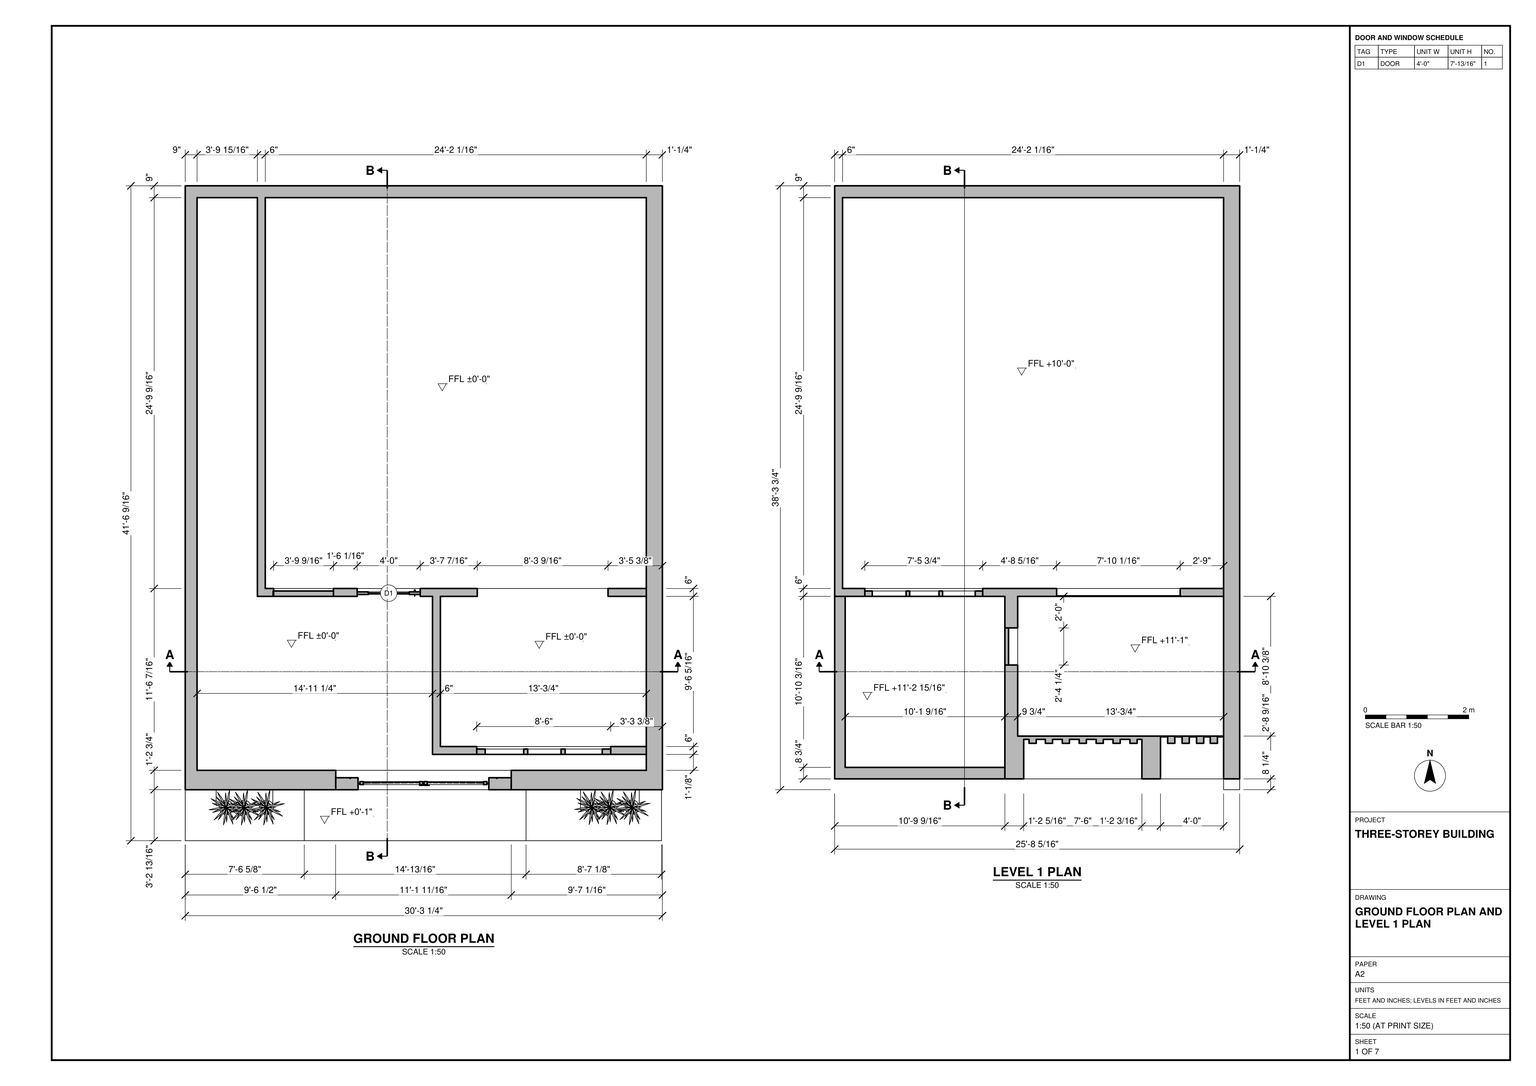
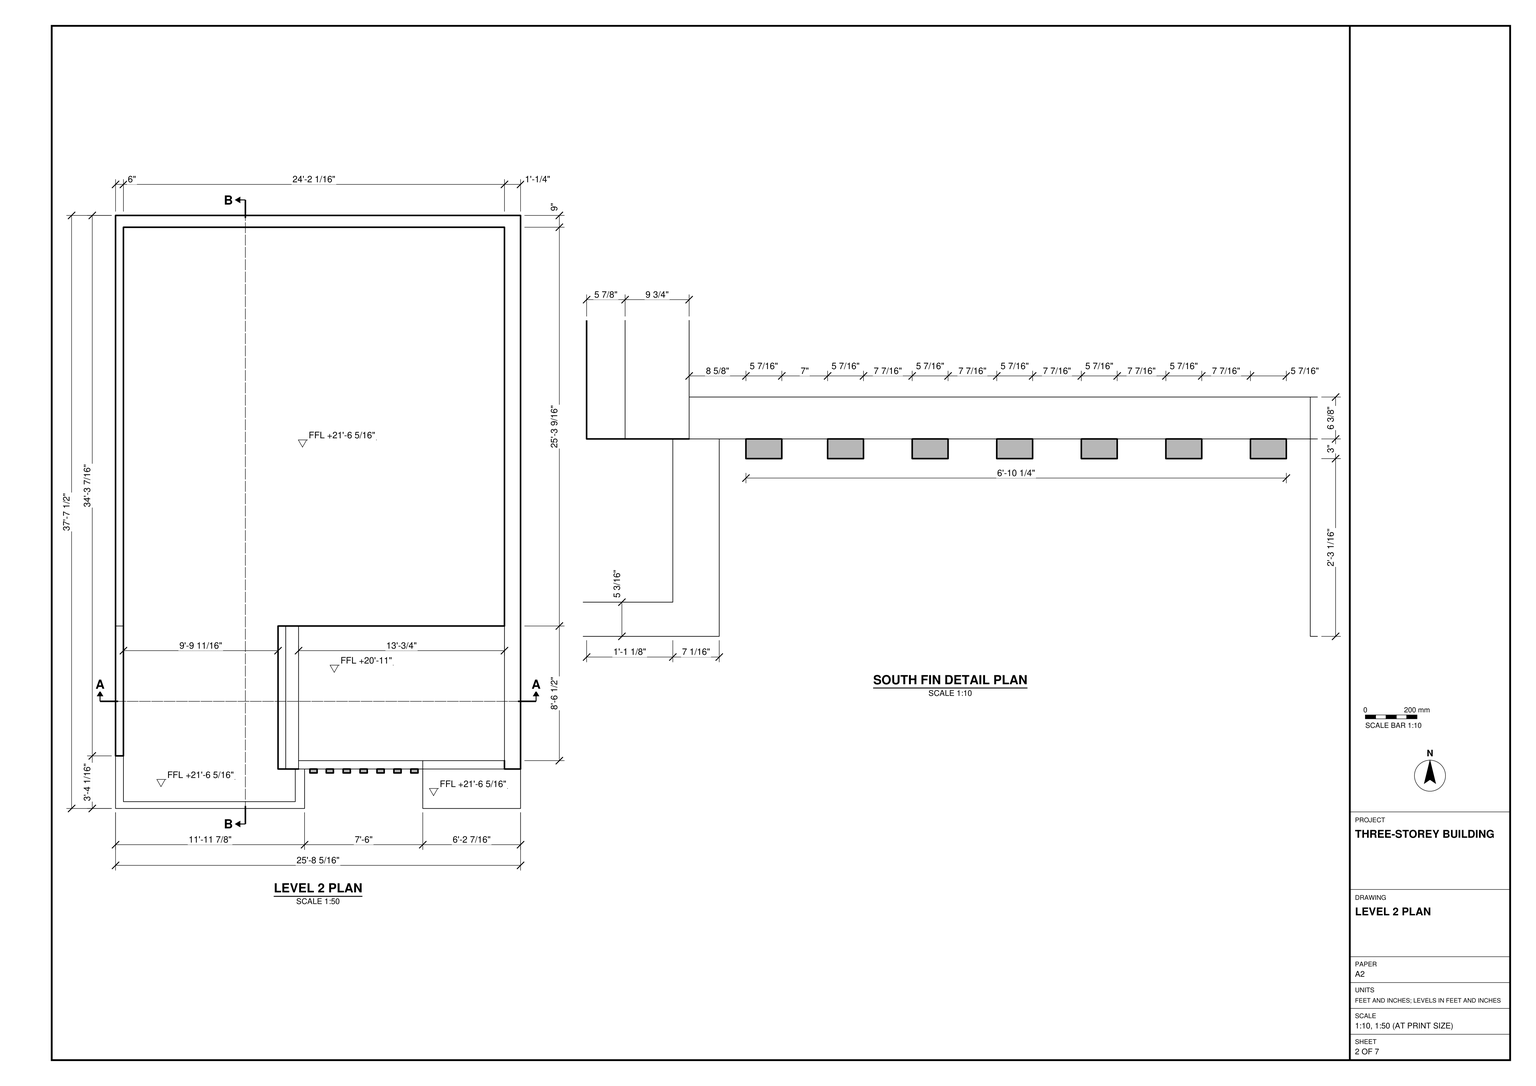
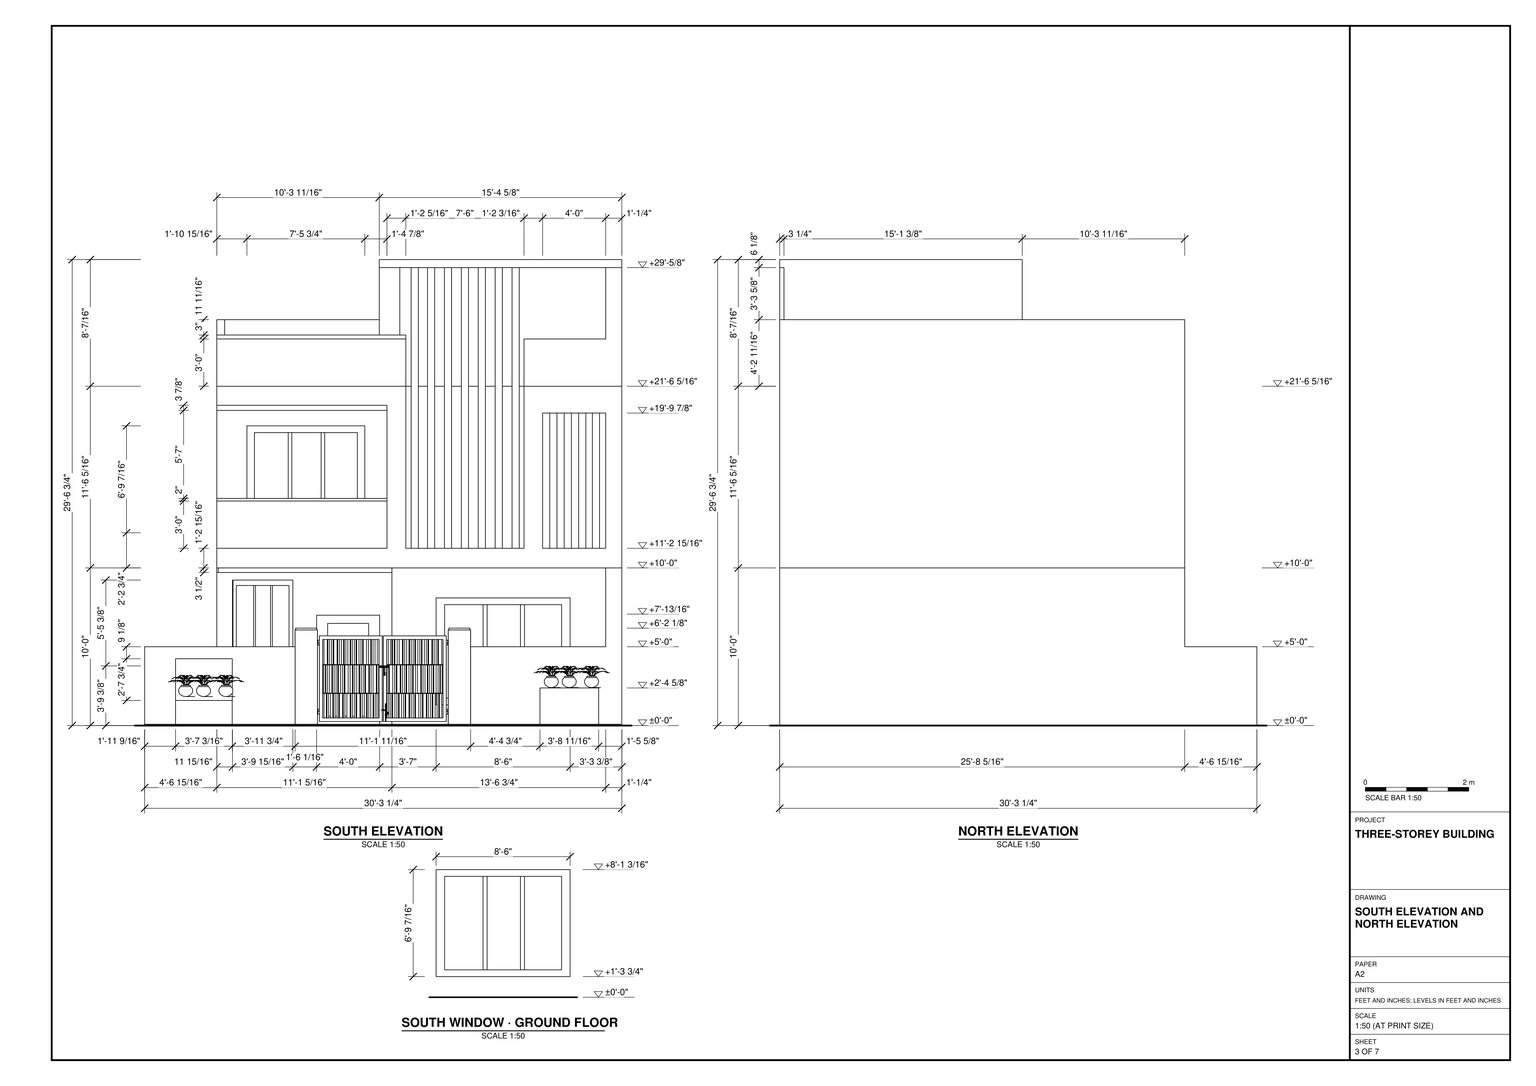
Build the three-storey building in SketchUp from task_files/diagram_01.pdf. Work in feet and inches. The overall model is 30'-3 1/4" wide, 41'-6 9/16" deep and 29'-6 3/4" high. Set the principal levels at ±0'-0", +10'-0" and +21'-6 5/16". Use the local floor levels on the plans for the areas that sit above or below these principal levels.

Lay out the ground-floor enclosure, including the narrow strip along the west side and the front room set back from the south boundary wall. Build the perimeter walls and partitions at their drawn thicknesses. Follow the upper plans for the narrower building footprint, floor slabs, roof and parapets. On the south face, place the framed openings behind the boundary wall and model the double-leaf entrance gate between its piers. Reproduce the recessed upper opening, the stepped roofline and the two fields of vertical fins. Use the fin detail plan to set the spacing and projection of the blades. Place the front planting on either side of the gate. Decor and loose items, including plants, may be any suitable library components.

Keep shell elements such as walls, slabs and roof, and each furniture or joinery piece shown, in separate groups or components. Use components for repeated parts. Save one SketchUp model as output_files/three_storey_building_with_a_finned_south_facade.skp.

# SketchUp Ruby script. Lengths in inches.
U = 1.inch
M = Sketchup.active_model
def pt(a) = Geom::Point3d.new(a.map { |v| v * U })
def face(e, loops, mat)
  f = e.add_face(loops[0].map { |a| pt(a) })
  loops[1..].each { |l| e.add_face(l.map { |a| pt(a) }).erase! }
  f.material = f.back_material = mat if mat
  f
end
# faces: each face lists its corners as indices into pts; further lists are holes
def faces(e, pts, list, mat = nil) = list.each { |f| face(e, (f[0].is_a?(Array) ? f : [f]).map { |l| l.map { |i| pts[i] } }, mat) }
# xy, xz, yz: faces in a plane at the given z, y or x. An outline is a flat list of corners, or four numbers for a rectangle; further outlines are holes
def ring(l) = l.size == 4 ? [[l[0], l[1]], [l[2], l[1]], [l[2], l[3]], [l[0], l[3]]] : l.each_slice(2).to_a
def flat(e, list, mat, &to3) = list.each { |f| face(e, (f[0].is_a?(Array) ? f : [f]).map { |l| ring(l).map { |u, v| to3.(u, v) } }, mat) }
def xy(e, z, list, mat = nil) = flat(e, list, mat) { |x, y| [x, y, z] }
def xz(e, y, list, mat = nil) = flat(e, list, mat) { |x, z| [x, y, z] }
def yz(e, x, list, mat = nil) = flat(e, list, mat) { |y, z| [x, y, z] }
def lines(e, pts, list) = list.each { |a, b| e.add_line(pt(pts[a]), pt(pts[b])) }
# prism: a flat outline (further loops are holes) pulled along v
def prism(e, loops, v, mat = nil)
  f = face(e, loops, mat); d = Geom::Vector3d.new(v.map { |x| x * U })
  f.pushpull(f.normal.samedirection?(d) ? d.length : -d.length)
end
def box(e, o, s, mat = nil) = prism(e, [[o, [o[0] + s[0], o[1], o[2]], [o[0] + s[0], o[1] + s[1], o[2]], [o[0], o[1] + s[1], o[2]]]], [0, 0, s[2]], mat)
def at(x, y, z, deg = 0) = Geom::Transformation.translation(pt([x, y, z])) * Geom::Transformation.rotation(ORIGIN, Z_AXIS, deg.degrees)
def axes(o, x, y, z) = Geom::Transformation.new([*x, 0, *y, 0, *z, 0, *pt(o).to_a, 1])
def part(name) = M.definitions.add(name)
# library, detail: a bought-in or finely detailed component or shape, given as its bounding box
def library(name, o, s) = part(name).tap { |d| box(d.entities, o, s) }
def detail(e, o, s) = box(e.add_group.entities, o, s)
def put(e, d, t, mat = nil) = e.add_instance(d, t).tap { |i| i.material = mat if mat }
def group(e, t, mat = nil) = e.add_group.tap { |g| g.transformation = t; g.material = mat if mat }.entities
root = M.entities
M.materials.add("3064d055d501e5e6b0f6546dbac280ca7b3e63756ead2-EpHpDy_fw4").color = [149, 120, 88]
M.materials.add("[Blacktop Old 02]").color = [143, 145, 145]
M.materials.add("[Blinds Roman Hobbled Blue]").color = [81, 82, 87]
M.materials.add("[Brick Tumbled]").color = [135, 132, 132]
M.materials.add("[Color C08]").color = [102, 51, 0]
M.materials.add("[Color H07]").color = [0, 153, 153]
M.materials.add("[Color L06]").color = [204, 0, 100]
M.materials.add("[Color L16]").color = [102, 0, 51]
M.materials.add("[Concrete Aggregate Smoke]").color = [154, 150, 148]
M.materials.add("[Concrete Form 4x8]").color = [167, 170, 168]
M.materials.add("[Grass Dark Green]").color = [106, 157, 55]
M.materials.add("[Metal Seamed]").color = [118, 119, 115]
M.materials.add("[Stone Flagstone Ashlar]").color = [175, 116, 102]
M.materials.add("[Translucent Glass Gray]").color = [128, 128, 128]
M.materials["[Translucent Glass Gray]"].alpha = 0.5
M.materials.add("[Wood Veneer 01]").color = [120, 70, 37]
c1 = library("Glass Door",[128.54,164.83,0],[40,4.88,84.84])
c2 = library("组\#1607",[0,0,0],[105.03,15.75,105.99])
c3 = part("组\#1597")
box(c3.entities,[0,0,0],[9.65,0.39,1.97])
box(c3.entities,[10.43,0,0],[1.58,0.39,1.97])
c4 = part("组\#1599")
prism(c4.entities,[[[0.05,0.59,0],[0.12,0.67,0],[0.2,0.73,0],[0.29,0.77,0],[0.39,0.79,0],[0.5,0.77,0],[0.59,0.73,0],[0.67,0.67,0],[0.73,0.59,0],[0.77,0.5,0],[0.79,0.39,0],[0.77,0.29,0],[0.73,0.2,0],[0.67,0.12,0],[0.59,0.05,0],[0.5,0.01,0],[0.39,0,0],[0.29,0.01,0],[0.2,0.05,0],[0.12,0.12,0],[0.05,0.2,0],[0.01,0.29,0],[0,0.39,0],[0.01,0.5,0]]],[0,0,12.4])
c5 = part("组\#1598")
prism(c5.entities,[[[-0.39,1.18,0.59],[-0.39,1.16,0.4375],[-0.39,1.1,0.3],[-0.39,1.01,0.17],[-0.39,0.89,0.08],[-0.39,0.74,0.02],[-0.39,0.59,0],[-0.39,0.4375,0.02],[-0.39,0.3,0.08],[-0.39,0.17,0.17],[-0.39,0.08,0.3],[-0.39,0.02,0.4375],[-0.39,0,0.59],[-0.39,0.02,0.74],[-0.39,0.08,0.89],[-0.39,0.17,1.01],[-0.39,0.3,1.1],[-0.39,0.4375,1.16],[-0.39,0.59,1.18],[-0.39,0.74,1.16],[-0.39,0.89,1.1],[-0.39,1.01,1.01],[-0.39,1.1,0.89],[-0.39,1.16,0.74]],[[-0.39,0.98,0.59],[-0.39,0.97,0.69],[-0.39,0.93,0.79],[-0.39,0.87,0.87],[-0.39,0.79,0.93],[-0.39,0.69,0.97],[-0.39,0.59,0.98],[-0.39,0.49,0.97],[-0.39,0.39,0.93],[-0.39,0.3125,0.87],[-0.39,0.25,0.79],[-0.39,0.21,0.69],[-0.39,0.2,0.59],[-0.39,0.21,0.49],[-0.39,0.25,0.39],[-0.39,0.3125,0.3125],[-0.39,0.39,0.25],[-0.39,0.49,0.21],[-0.39,0.59,0.2],[-0.39,0.69,0.21],[-0.39,0.79,0.25],[-0.39,0.87,0.3125],[-0.39,0.93,0.39],[-0.39,0.97,0.49]]],[1.97,0,0])
c6 = part("组\#1600")
prism(c6.entities,[[[0,1.18,0.59],[0,1.16,0.4375],[0,1.1,0.3],[0,1.01,0.17],[0,0.89,0.08],[0,0.74,0.02],[0,0.59,0],[0,0.4375,0.02],[0,0.3,0.08],[0,0.17,0.17],[0,0.08,0.3],[0,0.02,0.4375],[0,0,0.59],[0,0.02,0.74],[0,0.08,0.89],[0,0.17,1.01],[0,0.3,1.1],[0,0.4375,1.16],[0,0.59,1.18],[0,0.74,1.16],[0,0.89,1.1],[0,1.01,1.01],[0,1.1,0.89],[0,1.16,0.74]],[[0,0.98,0.59],[0,0.97,0.69],[0,0.93,0.79],[0,0.87,0.87],[0,0.79,0.93],[0,0.69,0.97],[0,0.59,0.98],[0,0.49,0.97],[0,0.39,0.93],[0,0.3125,0.87],[0,0.25,0.79],[0,0.21,0.69],[0,0.2,0.59],[0,0.21,0.49],[0,0.25,0.39],[0,0.3125,0.3125],[0,0.39,0.25],[0,0.49,0.21],[0,0.59,0.2],[0,0.69,0.21],[0,0.79,0.25],[0,0.87,0.3125],[0,0.93,0.39],[0,0.97,0.49]]],[1.18,0,0])
c7 = part("组\#1601")
prism(c7.entities,[[[0,1.18,0.59],[0,1.16,0.4375],[0,1.1,0.3],[0,1.01,0.17],[0,0.89,0.08],[0,0.74,0.02],[0,0.59,0],[0,0.4375,0.02],[0,0.3,0.08],[0,0.17,0.17],[0,0.08,0.3],[0,0.02,0.4375],[0,0,0.59],[0,0.02,0.74],[0,0.08,0.89],[0,0.17,1.01],[0,0.3,1.1],[0,0.4375,1.16],[0,0.59,1.18],[0,0.74,1.16],[0,0.89,1.1],[0,1.01,1.01],[0,1.1,0.89],[0,1.16,0.74]],[[0,0.98,0.59],[0,0.97,0.69],[0,0.93,0.79],[0,0.87,0.87],[0,0.79,0.93],[0,0.69,0.97],[0,0.59,0.98],[0,0.49,0.97],[0,0.39,0.93],[0,0.3125,0.87],[0,0.25,0.79],[0,0.21,0.69],[0,0.2,0.59],[0,0.21,0.49],[0,0.25,0.39],[0,0.3125,0.3125],[0,0.39,0.25],[0,0.49,0.21],[0,0.59,0.2],[0,0.69,0.21],[0,0.79,0.25],[0,0.87,0.3125],[0,0.93,0.39],[0,0.97,0.49]]],[1.57,0,0])
c8 = part("组\#1591")
xy(c8.entities,0,[[0.12,0,1.0625,0.39]])
xy(c8.entities,0.39,[[0,0,1.18,0.39]])
xy(c8.entities,0.79,[[0.39,0,0.79,0.39]])
xy(c8.entities,2.36,[[0.39,0,0.79,0.39]])
xy(c8.entities,2.76,[[0,0,1.18,0.39]])
xy(c8.entities,9.84,[[0,0,1.18,0.39]])
xz(c8.entities,0,[[0.12,0,1.0625,0,1.18,0.12,1.18,0.39,0,0.39,0,0.12],[[0,0.39,1.18,2.76],[0.39,0.79,0.79,2.36]],[0,2.76,1.18,9.84]])
xz(c8.entities,0.39,[[0.12,0,0,0.12,0,0.39,1.18,0.39,1.18,0.12,1.0625,0],[[0,0.39,1.18,2.76],[0.39,0.79,0.79,2.36]],[0,2.76,1.18,9.84]])
yz(c8.entities,0,[[0,0.12,0.39,0.39],[0,0.39,0.39,2.76],[0,2.76,0.39,8.46],[0,8.46,0.39,9.06],[0,9.06,0.39,9.84]])
yz(c8.entities,0.39,[[0,0.79,0.39,2.36]])
yz(c8.entities,0.79,[[0,0.79,0.39,2.36]])
yz(c8.entities,1.18,[[0,0.12,0.39,0.39],[0,0.39,0.39,2.76],[0,2.76,0.39,8.46],[0,8.46,0.39,8.86],[0,8.86,0.39,9.84]])
p = [[0.12,0,0],[0,0,0.12],[0,0.39,0.12],[0.12,0.39,0],[1.18,0,0.12],[1.0625,0,0],
  [1.0625,0.39,0],[1.18,0.39,0.12]]
faces(c8.entities,p,[[0,1,2,3],[4,5,6,7]])
c9 = part("组\#1592")
xy(c9.entities,0,[[0,0.71,0.8,1.1],[0.8,0.71,1.98,1.1],[1.98,0.71,3.95,1.1]])
xy(c9.entities,0.39,[[1.19,-0.63,1.59,1.1]])
xy(c9.entities,1.97,[[1.19,-0.63,1.59,1.1]])
xy(c9.entities,2.36,[[0,0.71,0.8,1.1],[0.8,0.71,1.98,1.1],[1.98,0.71,3.95,1.1]])
xz(c9.entities,-0.63,[[1.19,0.39,1.59,1.97]])
xz(c9.entities,0.71,[[0,0,3.95,2.36]])
xz(c9.entities,1.1,[[0,0,0.8,2.36],[[0.8,0,1.98,2.36],[1.19,0.39,1.59,1.97]],[1.98,0,3.95,2.36]])
yz(c9.entities,0,[[0.71,0,1.1,2.36]])
yz(c9.entities,1.19,[[-0.63,0.39,1.1,1.97]])
yz(c9.entities,1.59,[[-0.63,0.39,1.1,1.97]])
yz(c9.entities,3.95,[[0.71,0,1.1,2.36]])
c10 = part("组\#1602")
put(c10.entities,c8,at(0.8,0.39,0))
put(c10.entities,c9,at(-0.04,0.43,0.39))
c11 = part("组\#1609")
put(c11.entities,c3,at(0,1.1875,8.46))
put(c11.entities,c4,axes([0,0.2,9.84],[0,0,-1],[0,1,0],[1,0,0]))
put(c11.entities,c5,at(8.07,0.01,8.86))
put(c11.entities,c6,at(1.77,0.01,8.86))
put(c11.entities,c7,at(10.43,0.01,8.86))
put(c11.entities,c10,at(5.7,0,-0.16))
c12 = part("组\#1604")
prism(c12.entities,[[[0.08,0.89,0],[0.17,1.01,0],[0.3,1.1,0],[0.4375,1.16,0],[0.59,1.18,0],[0.74,1.16,0],[0.89,1.1,0],[1.01,1.01,0],[1.1,0.89,0],[1.16,0.74,0],[1.18,0.59,0],[1.16,0.4375,0],[1.1,0.3,0],[1.01,0.17,0],[0.89,0.08,0],[0.74,0.02,0],[0.59,0,0],[0.4375,0.02,0],[0.3,0.08,0],[0.17,0.17,0],[0.08,0.3,0],[0.02,0.4375,0],[0,0.59,0],[0.02,0.74,0]],[[0.97,0.49,0],[0.98,0.59,0],[0.97,0.69,0],[0.93,0.79,0],[0.87,0.87,0],[0.79,0.93,0],[0.69,0.97,0],[0.59,0.98,0],[0.49,0.97,0],[0.39,0.93,0],[0.3125,0.87,0],[0.25,0.79,0],[0.21,0.69,0],[0.2,0.59,0],[0.21,0.49,0],[0.25,0.39,0],[0.3125,0.3125,0],[0.39,0.25,0],[0.49,0.21,0],[0.59,0.2,0],[0.69,0.21,0],[0.79,0.25,0],[0.87,0.3125,0],[0.93,0.39,0]]],[0,0,3.9375])
c13 = part("组\#1603")
prism(c13.entities,[[[0.12,0.67,0],[0.2,0.73,0],[0.29,0.77,0],[0.39,0.79,0],[0.5,0.77,0],[0.59,0.73,0],[0.67,0.67,0],[0.73,0.59,0],[0.77,0.5,0],[0.79,0.39,0],[0.77,0.29,0],[0.73,0.2,0],[0.67,0.12,0],[0.59,0.05,0],[0.5,0.01,0],[0.39,0,0],[0.29,0.01,0],[0.2,0.05,0],[0.12,0.12,0],[0.05,0.2,0],[0.01,0.29,0],[0,0.39,0],[0.01,0.5,0],[0.05,0.59,0]]],[0,0,19.69])
c14 = part("组\#1606")
xy(c14.entities,0,[[2.95,0,4.13,0.39]])
xy(c14.entities,0.2,[[0,0,2.95,0.39],[2.95,0,4.13,0.39],[4.13,0,4.72,0.39]])
xy(c14.entities,0.6875,[[1.77,0,2.95,0.39]])
xy(c14.entities,0.89,[[1.77,0,2.95,0.39]])
xy(c14.entities,1.38,[[0,0,4.72,0.39]])
xz(c14.entities,0,[[2.95,0,4.13,0.2],[[0,0.2,4.72,1.38],[1.77,0.6875,2.95,0.89]]])
xz(c14.entities,0.39,[[2.95,0,4.13,0.2],[[0,0.2,4.72,1.38],[1.77,0.6875,2.95,0.89]]])
yz(c14.entities,0,[[0,0.2,0.39,1.38]])
yz(c14.entities,1.77,[[0,0.6875,0.39,0.89]])
yz(c14.entities,2.95,[[0,0,0.39,0.2],[0,0.6875,0.39,0.89]])
yz(c14.entities,4.13,[[0,0,0.39,0.2]])
yz(c14.entities,4.72,[[0,0.2,0.39,1.38]])
c15 = part("组\#1557")
xy(c15.entities,0,[[0,0,1.38,0.24]])
xy(c15.entities,1.18,[[0,0,0.19,0.24],[0.19,0,0.39,0.24],[0.39,0,0.99,0.24],[0.99,0,1.1875,0.24],[1.1875,0,1.38,0.24]])
xy(c15.entities,2.24,[[0.59,0,0.61,0.24],[0.77,0,0.79,0.24]])
xy(c15.entities,2.25,[[0.63,0,0.65,0.24],[0.65,0,0.68,0.24],[0.68,0,0.7,0.24],[0.7,0,0.72,0.24],[0.72,0,0.74,0.24]])
xy(c15.entities,2.45,[[0.65,0,0.6875,0.24],[0.6875,0,0.72,0.24]])
xz(c15.entities,0,[[0,0,1.38,1.18],[0.19,1.18,0.39,1.18,0.39,2.07,0.41,2.11,0.42,2.125,0.4375,2.14,0.45,2.16,0.47,2.17,0.49,2.1875,0.51,2.2,0.59,2.24,0.61,2.24,0.63,2.25,0.74,2.25,0.77,2.24,0.79,2.24,0.87,2.2,0.89,2.1875,0.91,2.18,0.92,2.16,0.9375,2.14,0.95,2.13,0.97,2.11,0.99,2.07,0.99,1.18,1.1875,1.18,1.1875,2.11,1.17,2.14,1.16,2.17,1.14,2.21,1.12,2.23,1.1,2.26,1.07,2.29,1.05,2.3125,1.02,2.34,0.99,2.36,0.93,2.39,0.9,2.41,0.86,2.42,0.83,2.43,0.8,2.4375,0.76,2.44,0.72,2.45,0.65,2.45,0.62,2.44,0.58,2.4375,0.51,2.42,0.48,2.41,0.45,2.39,0.39,2.36,0.36,2.34,0.33,2.3125,0.31,2.29,0.28,2.26,0.26,2.23,0.24,2.21,0.22,2.17,0.2,2.14,0.19,2.11]])
xz(c15.entities,0.24,[[0,0,1.38,1.18],[0.19,1.18,0.19,2.11,0.2,2.14,0.22,2.17,0.24,2.21,0.26,2.23,0.28,2.26,0.31,2.29,0.33,2.3125,0.36,2.34,0.39,2.36,0.45,2.39,0.48,2.41,0.51,2.42,0.58,2.4375,0.62,2.44,0.65,2.45,0.72,2.45,0.76,2.44,0.8,2.4375,0.83,2.43,0.86,2.42,0.9,2.41,0.93,2.39,0.99,2.36,1.02,2.34,1.05,2.3125,1.07,2.29,1.1,2.26,1.12,2.23,1.14,2.21,1.16,2.17,1.17,2.14,1.1875,2.11,1.1875,1.18,0.99,1.18,0.99,2.07,0.97,2.11,0.95,2.13,0.9375,2.14,0.92,2.16,0.91,2.18,0.89,2.1875,0.87,2.2,0.79,2.24,0.77,2.24,0.74,2.25,0.63,2.25,0.61,2.24,0.59,2.24,0.51,2.2,0.49,2.1875,0.47,2.17,0.45,2.16,0.4375,2.14,0.42,2.125,0.41,2.11,0.39,2.07,0.39,1.18]])
yz(c15.entities,0,[[0,0,0.24,1.18]])
yz(c15.entities,0.19,[[0,1.18,0.24,2.11]])
yz(c15.entities,0.39,[[0,1.18,0.24,2.07]])
yz(c15.entities,0.99,[[0,1.18,0.24,2.07]])
yz(c15.entities,1.1875,[[0,1.18,0.24,2.11]])
yz(c15.entities,1.38,[[0,0,0.24,1.18]])
p = [[0.19,0,2.11],[0.2,0,2.14],[0.2,0.24,2.14],[0.19,0.24,2.11],[0.22,0,2.17],[0.22,0.24,2.17],
  [0.45,0,2.16],[0.4375,0,2.14],[0.4375,0.24,2.14],[0.45,0.24,2.16],[0.42,0,2.125],[0.42,0.24,2.125],
  [0.41,0,2.11],[0.41,0.24,2.11],[0.4,0,2.09],[0.4,0.24,2.09],[0.39,0,2.07],[0.39,0.24,2.07],
  [0.95,0,2.13],[0.9375,0,2.14],[0.9375,0.24,2.14],[0.95,0.24,2.13],[0.92,0,2.16],[0.92,0.24,2.16],
  [0.99,0,2.07],[0.97,0,2.11],[0.97,0.24,2.11],[0.99,0.24,2.07],[1.16,0,2.17],[1.17,0,2.14],
  [1.17,0.24,2.14],[1.16,0.24,2.17],[1.1875,0,2.11],[1.1875,0.24,2.11],[0.24,0,2.21],[0.24,0.24,2.21],
  [0.26,0,2.23],[0.26,0.24,2.23],[0.28,0,2.26],[0.28,0.24,2.26],[0.57,0,2.23],[0.55,0,2.22],
  [0.55,0.24,2.22],[0.57,0.24,2.23],[0.53,0,2.21],[0.53,0.24,2.21],[0.51,0,2.2],[0.51,0.24,2.2],
  [0.49,0,2.1875],[0.49,0.24,2.1875],[0.47,0,2.17],[0.47,0.24,2.17],[0.63,0,2.25],[0.61,0,2.24],
  [0.61,0.24,2.24],[0.63,0.24,2.25],[0.59,0,2.24],[0.59,0.24,2.24],[0.77,0,2.24],[0.74,0,2.25],
  [0.74,0.24,2.25],[0.77,0.24,2.24],[0.87,0,2.2],[0.85,0,2.21],[0.85,0.24,2.21],[0.87,0.24,2.2],
  [0.83,0,2.22],[0.83,0.24,2.22],[0.81,0,2.23],[0.81,0.24,2.23],[0.79,0,2.24],[0.79,0.24,2.24],
  [0.91,0,2.18],[0.91,0.24,2.18],[0.89,0,2.1875],[0.89,0.24,2.1875],[1.1,0,2.26],[1.12,0,2.23],
  [1.12,0.24,2.23],[1.1,0.24,2.26],[1.14,0,2.21],[1.14,0.24,2.21],[0.31,0,2.29],[0.31,0.24,2.29],
  [0.33,0,2.3125],[0.33,0.24,2.3125],[0.36,0,2.34],[0.36,0.24,2.34],[0.39,0,2.36],[0.39,0.24,2.36],
  [0.99,0,2.36],[1.02,0,2.34],[1.02,0.24,2.34],[0.99,0.24,2.36],[1.05,0,2.3125],[1.05,0.24,2.3125],
  [1.07,0,2.29],[1.07,0.24,2.29],[0.42,0,2.375],[0.42,0.24,2.375],[0.45,0,2.39],[0.45,0.24,2.39],
  [0.48,0,2.41],[0.48,0.24,2.41],[0.51,0,2.42],[0.51,0.24,2.42],[0.55,0,2.43],[0.55,0.24,2.43],
  [0.58,0,2.4375],[0.58,0.24,2.4375],[0.62,0,2.44],[0.62,0.24,2.44],[0.65,0,2.45],[0.65,0.24,2.45],
  [0.72,0,2.45],[0.76,0,2.44],[0.76,0.24,2.44],[0.72,0.24,2.45],[0.8,0,2.4375],[0.8,0.24,2.4375],
  [0.83,0,2.43],[0.83,0.24,2.43],[0.86,0,2.42],[0.86,0.24,2.42],[0.9,0,2.41],[0.9,0.24,2.41],
  [0.93,0,2.39],[0.93,0.24,2.39],[0.96,0,2.375],[0.96,0.24,2.375]]
faces(c15.entities,p,[[0,1,2,3],[1,4,5,2],[6,7,8,9],[7,10,11,8],[10,12,13,11],[12,14,15,13],[14,16,17,15],[18,19,20,21],
  [19,22,23,20],[24,25,26,27],[25,18,21,26],[28,29,30,31],[29,32,33,30],[4,34,35,5],[34,36,37,35],[36,38,39,37],
  [40,41,42,43],[41,44,45,42],[44,46,47,45],[46,48,49,47],[48,50,51,49],[50,6,9,51],[52,53,54,55],[56,40,43,57],
  [58,59,60,61],[62,63,64,65],[63,66,67,64],[66,68,69,67],[68,70,71,69],[22,72,73,23],[72,74,75,73],[74,62,65,75],
  [76,77,78,79],[77,80,81,78],[80,28,31,81],[38,82,83,39],[82,84,85,83],[84,86,87,85],[86,88,89,87],[90,91,92,93],
  [91,94,95,92],[94,96,97,95],[96,76,79,97],[88,98,99,89],[98,100,101,99],[100,102,103,101],[102,104,105,103],[104,106,107,105],
  [106,108,109,107],[108,110,111,109],[110,112,113,111],[114,115,116,117],[115,118,119,116],[118,120,121,119],[120,122,123,121],[122,124,125,123],
  [124,126,127,125],[126,128,129,127],[128,90,93,129]])
c16 = part("组\#1593")
xy(c16.entities,1.4,[[0.2,0.43,3.35,0.71]])
xy(c16.entities,1.89,[[1.77,0,2.95,0.43],[1.77,0.43,2.95,0.71],[1.77,0.71,2.95,1.05]])
xy(c16.entities,2.09,[[1.77,0,2.95,0.43],[1.77,0.43,2.95,0.71],[1.77,0.71,2.95,1.05]])
xy(c16.entities,2.58,[[0,0.43,3.35,0.71]])
xz(c16.entities,0,[[1.77,1.89,2.95,2.09]])
xz(c16.entities,0.43,[[[0,1.4,3.35,2.58],[1.77,1.89,2.95,2.09]]])
xz(c16.entities,0.71,[[[0,1.4,3.35,2.58],[1.77,1.89,2.95,2.09]]])
xz(c16.entities,1.05,[[1.77,1.89,2.95,2.09]])
yz(c16.entities,1.77,[[0,1.89,0.43,2.09],[0.43,1.89,0.71,2.09],[0.71,1.89,1.05,2.09]])
yz(c16.entities,2.95,[[0,1.89,0.43,2.09],[0.43,1.89,0.71,2.09],[0.71,1.89,1.05,2.09]])
yz(c16.entities,3.35,[[0.43,1.4,0.71,2.58]])
p = [[0,0.31,2.58],[0,0.43,2.58],[0,0.31,1.4],[0,0.43,1.4],[0.2,0.31,1.4],[0.2,0.43,1.4]]
lines(c16.entities,p,[[0,1],[2,3],[4,5]])
put(c16.entities,c15,at(1.27,0.04,0))
c17 = part("组\#1605")
xy(c17.entities,1.4,[[0,0.31,0.2,0.71]])
yz(c17.entities,0,[[0.31,1.4,0.71,2.58]])
put(c17.entities,c16,at(0,0,0))
c18 = part("组\#1608")
put(c18.entities,c12,at(4.41,0,5.12))
put(c18.entities,c13,at(4.61,0.2,0))
put(c18.entities,c14,at(0,0.35,11.8125))
put(c18.entities,c12,at(4.41,0,14.96))
put(c18.entities,c17,at(5.35,0.09,7.63))
c19 = part("Main Gate")
put(c19.entities,c2,axes([15.75,105.03,0],[0.00003,-1,0],[-1,-0.00003,0],[0,0,1]),"3064d055d501e5e6b0f6546dbac280ca7b3e63756ead2-EpHpDy_fw4")
put(c19.entities,c2,at(15.75,106.3,0,90.002),"3064d055d501e5e6b0f6546dbac280ca7b3e63756ead2-EpHpDy_fw4")
put(c19.entities,c11,at(5.13,110.73,54.04,-89.998),"3064d055d501e5e6b0f6546dbac280ca7b3e63756ead2-EpHpDy_fw4")
put(c19.entities,c18,at(5.57,107.19,3.1,-89.998),"3064d055d501e5e6b0f6546dbac280ca7b3e63756ead2-EpHpDy_fw4")
c20 = part("Group\#1")
xy(c20.entities,0,[[0,0,59.8125,6]],"[Color C08]")
xy(c20.entities,3.79,[[20.96,0,22.77,6],[37.65,0,39.46,6]])
xy(c20.entities,3.79,[[3.79,0,20.96,6],[22.77,0,37.65,6],[39.46,0,56.03,6]],"[Color C08]")
xy(c20.entities,56.03,[[20.96,0,22.77,6],[37.65,0,39.46,6]])
xy(c20.entities,56.03,[[3.79,0,20.96,6],[22.77,0,37.65,6],[39.46,0,56.03,6]],"[Color C08]")
xy(c20.entities,59.8125,[[0,0,59.8125,6]],"[Color C08]")
xz(c20.entities,0,[[[0,0,59.8125,59.8125],[3.79,3.79,56.03,56.03]],[20.96,3.79,22.77,56.03],[37.65,3.79,39.46,56.03]],"[Color C08]")
xz(c20.entities,0,[[3.79,3.79,20.96,56.03],[22.77,3.79,37.65,56.03],[39.46,3.79,56.03,56.03]],"[Translucent Glass Gray]")
xz(c20.entities,6,[[[0,0,59.8125,59.8125],[3.79,3.79,56.03,56.03]],[20.96,3.79,22.77,56.03],[37.65,3.79,39.46,56.03]],"[Color C08]")
yz(c20.entities,0,[[0,0,6,59.8125]],"[Color C08]")
yz(c20.entities,3.79,[[0,3.79,6,56.03]],"[Color C08]")
yz(c20.entities,20.96,[[0,3.79,6,56.03]],"[Color C08]")
yz(c20.entities,22.77,[[0,3.79,6,56.03]],"[Color C08]")
yz(c20.entities,37.65,[[0,3.79,6,56.03]],"[Color C08]")
yz(c20.entities,39.46,[[0,3.79,6,56.03]],"[Color C08]")
yz(c20.entities,56.03,[[0,3.79,6,56.03]],"[Color C08]")
yz(c20.entities,59.8125,[[0,0,6,59.8125]],"[Color C08]")
c21 = part("Group\#2")
xy(c21.entities,0,[[0,0,6,43.6875]],"[Color C08]")
xy(c21.entities,3.05,[[0,3.05,6,40.64]],"[Color C08]")
xy(c21.entities,40.64,[[0,3.05,6,40.64]],"[Color C08]")
xy(c21.entities,43.6875,[[0,0,6,43.6875]],"[Color C08]")
xz(c21.entities,0,[[0,0,6,43.6875]],"[Color C08]")
xz(c21.entities,3.05,[[0,3.05,6,40.64]],"[Color C08]")
xz(c21.entities,40.64,[[0,3.05,6,40.64]],"[Color C08]")
xz(c21.entities,43.6875,[[0,0,6,43.6875]],"[Color C08]")
yz(c21.entities,0,[[[0,0,43.6875,43.6875],[3.05,3.05,40.64,40.64]]],"[Color C08]")
yz(c21.entities,0,[[3.05,3.05,40.64,40.64]],"[Translucent Glass Gray]")
yz(c21.entities,6,[[[0,0,43.6875,43.6875],[3.05,3.05,40.64,40.64]]],"[Color C08]")
c22 = library("Group\#139",[0,0,0],[57.47,26.82,16.2])
xy(root,0,[[0,0,0,38.8125,23.55,38.8125,23.55,26.8125,66.67,26.8125,66.67,38.8125,362.5625,38.8125,362.5625,0],[23.55,26.8125,66.67,38.8125],[0,38.8125,0,498.5625,54.9375,498.5625,54.9375,489.5625,9,489.5625,9,38.8125],[9,38.8125,188.25,53.5625],[351,38.8125,351,489.5625,54.9375,489.5625,54.9375,498.5625,363.25,498.5625,363.25,38.8125],
  [188.25,38.8125,351,53.5625],[188.25,65.6875,188.25,186,178.91,186,178.91,192,222.32,192,222.32,186,194.25,186,194.25,71.6875,351,71.6875,351,65.6875],[194.25,71.6875,351,71.6875,351,186,321.87,186,321.87,192,222.32,192,222.32,186,194.25,186],[54.9375,186,54.9375,489.5625,60.9375,489.5625,60.9375,192,130.91,192,130.91,186],[321.87,186,351,192],
  [60.9375,192,351,489.5625]])
xy(root,0,[[9,53.5625,351,53.5625,351,65.6875,188.25,65.6875,188.25,186,178.91,186,178.91,192,130.91,192,130.91,186,54.9375,186,54.9375,489.5625,9,489.5625]],"[Concrete Aggregate Smoke]")
xy(root,0.875,[[114.58,38.8125,248.18,53.5625]])
xy(root,1,[[300.94,23.375,345.64,38.8125]])
xy(root,1,[[90.625,0,259.45,38.8125]],"[Concrete Form 4x8]")
xy(root,1,[[0,0,90.625,0,90.625,38.8125,66.67,38.8125,66.67,26.8125,23.55,26.8125,23.55,38.8125,0,38.8125],[259.45,0,362.5625,0,362.5625,38.8125,345.64,38.8125,345.64,23.375,300.94,23.375,300.94,38.8125,259.45,38.8125]],"[Grass Dark Green]")
xy(root,15.75,[[221.9,65.6875,323.9,71.6875]])
xy(root,19.11,[[23.55,26.8125,66.67,38.8125]],"[Brick Tumbled]")
xy(root,28.625,[[300.94,23.375,345.64,38.8125]],"[Brick Tumbled]")
xy(root,45.39,[[67.29,186,112.85,192]])
xy(root,54.6,[[188.25,110.11,194.25,147.92]])
xy(root,60,[[0,38.8125,114.58,38.8125,114.58,53.5625,9,53.5625,9,489.5625,54.9375,489.5625,54.9375,498.5625,0,498.5625],[248.18,38.8125,351,53.5625]],"[Stone Flagstone Ashlar]")
xy(root,84,[[130.91,186,178.91,192]])
xy(root,97.18,[[221.9,65.6875,323.9,71.6875]])
xy(root,101.16,[[188.25,110.11,194.25,147.92]])
xy(root,107.13,[[222.32,186,321.87,192]])
xy(root,110.77,[[67.29,186,112.85,192]])
xy(root,116.5,[[56.0625,52.5,188.25,186]],"[Wood Veneer 01]")
xy(root,120,[[351,38.8125,363.25,47.0625],[56.0625,52.5,188.25,186],[54.9375,65.6875,56.0625,67.1875],[54.9375,67.1875,56.0625,186],[60.9375,192,351,489.5625]])
xy(root,120,[[54.9375,47.0625,54.9375,65.6875,56.0625,65.6875,56.0625,52.5,188.25,52.5,188.25,65.6875,351,65.6875,351,47.0625]],"[Color L16]")
xy(root,129,[[194.25,71.6875,351,79.625],[194.25,79.625,351,186],[223.9,186,317.97,192]])
xy(root,133,[[194.25,79.625,351,186],[223.9,186,317.97,186.375]])
xy(root,134.9375,[[54.9375,47.0625,54.9375,186,62.93,186,62.93,55.8,184.5,55.8,184.5,47.0625],[62.93,55.8,184.5,186],[184.5,65.6875,188.25,77.125],[308.41,74.125,313.875,79.0625],[184.5,77.125,188.25,186]])
xy(root,134.9375,[[198.83,47.0625,288.82,47.0625,288.82,77.125,285.17,77.125,285.17,74.125,279.71,74.125,279.71,77.125,272.3,77.125,272.3,74.125,266.83,74.125,266.83,77.125,259.42,77.125,259.42,74.125,253.96,74.125,253.96,77.125,246.55,77.125,246.55,74.125,241.08,74.125,241.08,77.125,233.67,77.125,233.67,74.125,228.21,74.125,228.21,77.125,220.8,77.125,220.8,74.125,215.33,74.125,215.33,77.125,208.36,77.125,208.36,74.125,202.9,74.125,202.9,77.125,198.83,77.125],[302.98,47.0625,351,47.0625,351,79.0625,346.3125,79.0625,346.3125,74.125,340.85,74.125,340.85,79.0625,335.875,79.0625,335.875,74.125,330.41,74.125,330.41,79.0625,324.875,79.0625,324.875,74.125,319.41,74.125,319.41,79.0625,313.875,79.0625,313.875,74.125,308.41,74.125,308.41,79.0625,302.98,79.0625]],"[Color H07]")
xy(root,147.65,[[77.88,186,167.61,192]])
xy(root,164.71,[[184.5,133.73,194.25,161.98]])
xy(root,170.9375,[[54.9375,47.0625,54.9375,186,62.93,186,62.93,55.8,184.5,55.8,184.5,47.0625]])
xy(root,172.9375,[[54.9375,47.0625,184.5,47.0625,184.5,55.8,62.93,55.8,62.93,186,54.9375,186]],"[Metal Seamed]")
xy(root,228.1875,[[77.88,186,167.61,192]])
xy(root,229.46,[[184.5,133.73,194.25,161.98]])
xy(root,230.7,[[223.9,186,317.97,186.375],[223.9,186.375,317.97,192]])
xy(root,237.89,[[308.41,74.125,313.875,79.0625]])
xy(root,237.89,[[302.98,47.0625,302.98,79.0625,308.41,79.0625,308.41,74.125,313.875,74.125,313.875,79.0625,319.41,79.0625,319.41,74.125,324.875,74.125,324.875,79.0625,330.41,79.0625,330.41,74.125,335.875,74.125,335.875,79.0625,340.85,79.0625,340.85,74.125,346.3125,74.125,346.3125,79.0625,351,79.0625,351,47.0625]],"[Color H07]")
xy(root,239.9375,[[54.9375,47.0625,184.5,186]],"[Wood Veneer 01]")
xy(root,243.8125,[[54.9375,47.0625,184.5,186]],"[Concrete Aggregate Smoke]")
xy(root,249,[[194.25,79.625,351,186]])
xy(root,251,[[194.25,79.625,351,186]],"[Concrete Aggregate Smoke]")
xy(root,258.3125,[[54.9375,47.0625,54.9375,87.125,60.9375,87.125,60.9375,52.27,191.76,52.27,191.76,77.125,198.83,77.125,198.83,47.0625],[288.82,77.125,351,83.5],[54.9375,87.125,60.9375,186]])
xy(root,258.3125,[[60.9375,52.27,191.76,52.27,191.76,77.125,178.64,77.125,178.64,186,351,186,351,489.5625,60.9375,489.5625]],"[Blacktop Old 02]")
xy(root,258.3125,[[288.82,47.0625,363.25,77.125]],"[Color H07]")
xy(root,258.3125,[[194.25,77.125,288.82,83.5]],"[Concrete Aggregate Smoke]")
xy(root,294.3125,[[54.9375,47.0625,54.9375,87.125,60.9375,87.125,60.9375,52.27,191.76,52.27,191.76,77.125,198.83,77.125,198.83,47.0625]])
xy(root,294.3125,[[288.82,77.125,351,83.5]],"[Color H07]")
xy(root,297.3125,[[54.9375,47.0625,198.83,47.0625,198.83,77.125,191.76,77.125,191.76,52.27,60.9375,52.27,60.9375,87.125,54.9375,87.125]],"[Metal Seamed]")
xy(root,309,[[54.9375,87.125,60.9375,87.125,60.9375,489.5625,351,489.5625,351,186,360,186,360,498.5625,54.9375,498.5625],[360,186,363.25,498.5625]],"[Color L06]")
xy(root,348.625,[[202.9,74.125,208.36,77.125],[215.33,74.125,220.8,77.125],[228.21,74.125,233.67,77.125],[241.08,74.125,246.55,77.125],[253.96,74.125,259.42,77.125],
  [266.83,74.125,272.3,77.125],[279.71,74.125,285.17,77.125]])
xy(root,348.625,[[178.64,74.125,194.25,77.125],[194.25,74.125,194.25,83.5,351,83.5,351,77.125,363.25,77.125,363.25,74.125,285.17,74.125,285.17,77.125,279.71,77.125,279.71,74.125,272.3,74.125,272.3,77.125,266.83,77.125,266.83,74.125,259.42,74.125,259.42,77.125,253.96,77.125,253.96,74.125,246.55,74.125,246.55,77.125,241.08,77.125,241.08,74.125,233.67,74.125,233.67,77.125,228.21,77.125,228.21,74.125,220.8,74.125,220.8,77.125,215.33,77.125,215.33,74.125,208.36,74.125,208.36,77.125,202.9,77.125,202.9,74.125],[360,77.125,363.25,186]],"[Color H07]")
xy(root,354.75,[[178.64,74.125,363.25,186]],"[Color H07]")
xz(root,0,[[0,0,362.5625,1]])
xz(root,23.375,[[300.94,1,345.64,28.625]],"[Brick Tumbled]")
xz(root,26.8125,[[23.55,0,66.67,1]])
xz(root,26.8125,[[23.55,1,66.67,19.11]],"[Brick Tumbled]")
xz(root,38.8125,[[0,0,9,1],[9,0,23.55,1],[23.55,0,66.67,19.11],[66.67,0,188.25,0,188.25,0.875,114.58,0.875,114.58,1,66.67,1],[188.25,0,351,0,351,1,248.18,1,248.18,0.875,188.25,0.875],
  [351,0,362.5625,1],[114.58,0.875,188.25,1],[188.25,0.875,248.18,1],[300.94,1,345.64,28.625]])
xz(root,38.8125,[[23.55,19.11,66.73,50.86]],"[Blinds Roman Hobbled Blue]")
xz(root,38.8125,[[362.5625,0,363.25,0,363.25,120,351,120,351,60,248.18,60,248.18,1,300.94,1,300.94,28.625,345.64,28.625,345.64,1,362.5625,1],[0,1,23.55,1,23.55,50.86,66.73,50.86,66.73,19.11,66.67,19.11,66.67,1,114.58,1,114.58,60,0,60]],"[Stone Flagstone Ashlar]")
xz(root,47.0625,[[[54.9375,120,363.25,120,363.25,258.3125,288.82,258.3125,288.82,134.9375,198.83,134.9375,198.83,258.3125,54.9375,258.3125,54.9375,243.8125,184.5,243.8125,184.5,134.9375,54.9375,134.9375],[302.98,134.9375,351,237.89]]],"[Color H07]")
xz(root,47.0625,[[54.9375,170.9375,184.5,172.9375],[54.9375,294.3125,198.83,297.3125]],"[Metal Seamed]")
xz(root,47.0625,[[54.9375,134.9375,184.5,170.9375],[54.9375,258.3125,198.83,294.3125]],"[Translucent Glass Gray]")
xz(root,47.0625,[[54.9375,239.9375,184.5,243.8125]],"[Wood Veneer 01]")
xz(root,52.27,[[60.9375,294.3125,191.76,297.3125]],"[Metal Seamed]")
xz(root,52.27,[[60.9375,258.3125,191.76,294.3125]],"[Translucent Glass Gray]")
xz(root,52.5,[[56.0625,116.5,188.25,120]],"[Wood Veneer 01]")
xz(root,53.5625,[[9,0,9,60,114.58,60,114.58,0.875,248.18,0.875,248.18,60,351,60,351,0]],"[Stone Flagstone Ashlar]")
xz(root,55.8,[[62.93,170.9375,184.5,172.9375]],"[Metal Seamed]")
xz(root,55.8,[[62.93,134.9375,184.5,170.9375]],"[Translucent Glass Gray]")
xz(root,65.6875,[[[188.25,0,351,120],[221.9,15.75,323.9,97.18]]],"[Color L16]")
xz(root,71.6875,[[[194.25,0,351,120],[221.9,15.75,323.9,97.18]],[194.25,120,351,129]])
xz(root,74.125,[[178.64,348.625,363.25,354.75]],"[Color H07]")
xz(root,74.125,[[202.9,134.9375,208.36,348.625],[215.33,134.9375,220.8,348.625],[228.21,134.9375,233.67,348.625],[241.08,134.9375,246.55,348.625],[253.96,134.9375,259.42,348.625],
  [266.83,134.9375,272.3,348.625],[279.71,134.9375,285.17,348.625],[308.41,134.9375,313.875,237.89],[319.41,134.9375,324.875,237.89],[330.41,134.9375,335.875,237.89],
  [340.85,134.9375,346.3125,237.89]],"[Wood Veneer 01]")
xz(root,77.125,[[194.25,249,198.83,258.3125],[202.9,249,208.36,258.3125],[215.33,249,220.8,258.3125],[228.21,249,233.67,258.3125],[241.08,249,246.55,258.3125],
  [253.96,249,259.42,258.3125],[266.83,249,272.3,258.3125],[279.71,249,285.17,258.3125],[288.82,249,351,258.3125],[191.76,258.3125,194.25,294.3125],
  [194.25,258.3125,198.83,294.3125],[202.9,258.3125,208.36,348.625],[215.33,258.3125,220.8,348.625],[228.21,258.3125,233.67,348.625],[241.08,258.3125,246.55,348.625],
  [253.96,258.3125,259.42,348.625],[266.83,258.3125,272.3,348.625],[279.71,258.3125,285.17,348.625],[191.76,294.3125,194.25,297.3125],[194.25,294.3125,198.83,297.3125]])
xz(root,77.125,[[178.64,258.3125,191.76,258.3125,191.76,297.3125,194.25,297.3125,194.25,348.625,178.64,348.625],[288.82,258.3125,363.25,258.3125,363.25,348.625,351,348.625,351,294.3125,288.82,294.3125]],"[Color H07]")
xz(root,77.125,[[198.83,134.9375,202.9,258.3125],[208.36,134.9375,215.33,258.3125],[220.8,134.9375,228.21,258.3125],[233.67,134.9375,241.08,258.3125],[246.55,134.9375,253.96,258.3125],
  [259.42,134.9375,266.83,258.3125],[272.3,134.9375,279.71,258.3125],[285.17,134.9375,288.82,258.3125]],"[Translucent Glass Gray]")
xz(root,79.0625,[[308.41,126.99,313.875,134.9375],[308.41,237.89,313.875,250.37]])
xz(root,79.0625,[[302.98,134.9375,308.41,237.89],[313.875,134.9375,319.41,237.89],[324.875,134.9375,330.41,237.89],[335.875,134.9375,340.85,237.89],[346.3125,134.9375,351,237.89]],"[Wood Veneer 01]")
xz(root,79.625,[[194.25,129,351,133],[194.25,133,351,249],[194.25,249,351,251]])
xz(root,83.5,[[288.82,258.3125,351,294.3125]])
xz(root,87.125,[[54.9375,258.3125,60.9375,294.3125],[54.9375,294.3125,60.9375,297.3125]])
xz(root,87.125,[[54.9375,297.3125,60.9375,309]],"[Color L06]")
xz(root,110.11,[[188.25,54.6,194.25,101.16]])
xz(root,133.73,[[184.5,164.71,194.25,229.46]])
xz(root,147.92,[[188.25,54.6,194.25,101.16]])
xz(root,161.98,[[184.5,164.71,194.25,229.46]])
xz(root,186,[[194.25,0,222.32,0,222.32,107.13,321.87,107.13,321.87,0,351,0,351,120,194.25,120],[54.9375,116.5,56.0625,120],[56.0625,116.5,188.25,120],[194.25,120,351,129],[194.25,129,223.9,133],
  [223.9,129,317.97,133],[317.97,129,351,133],[194.25,133,223.9,133,223.9,230.7,317.97,230.7,317.97,133,351,133,351,249,194.25,249],[223.9,133,317.97,230.7],[54.9375,134.9375,62.93,170.9375],
  [54.9375,170.9375,62.93,172.9375],[54.9375,239.9375,184.5,243.8125],[194.25,249,328.46,251],[328.46,249,338.4,251],[338.4,249,351,251]])
xz(root,186,[[360,309,363.25,348.625]],"[Color H07]")
xz(root,186,[[[54.9375,0,130.91,0,130.91,84,178.91,84,178.91,0,188.25,0,188.25,116.5,54.9375,116.5],[67.29,45.39,112.85,110.77]],[[62.93,134.9375,184.5,134.9375,184.5,239.9375,54.9375,239.9375,54.9375,172.9375,62.93,172.9375],[77.88,147.65,167.61,228.1875]]],"[Color L06]")
xz(root,186,[[194.25,251,351,258.3125]],"[Concrete Aggregate Smoke]")
xz(root,186,[[178.64,258.3125,178.64,354.75,363.25,354.75,363.25,348.625,360,348.625,360,309,351,309,351,258.3125]],"[Translucent Glass Gray]")
xz(root,186.375,[[223.9,133,317.97,230.7]])
xz(root,192,[[[60.9375,0,60.9375,120,351,120,351,0,321.87,0,321.87,107.13,222.32,107.13,222.32,0,178.91,0,178.91,84,130.91,84,130.91,0],[67.29,45.39,112.85,110.77]],[[60.9375,120,351,249],[223.9,129,317.97,230.7],[77.88,147.65,167.61,228.1875]]])
xz(root,489.5625,[[60.9375,0,351,120],[60.9375,120,351,249],[60.9375,249,89.1875,258.3125],[89.1875,249,351,258.3125]])
xz(root,489.5625,[[60.9375,258.3125,351,309]],"[Color L06]")
xz(root,489.5625,[[9,0,54.9375,60]],"[Stone Flagstone Ashlar]")
xz(root,498.5625,[[0,0,0,60,54.9375,60,54.9375,120,363.25,120,363.25,0],[54.9375,120,363.25,309]],"[Color L06]")
yz(root,0,[[0,0,38.8125,1]])
yz(root,0,[[38.8125,0,498.5625,60]],"[Stone Flagstone Ashlar]")
yz(root,9,[[53.5625,0,489.5625,60]],"[Stone Flagstone Ashlar]")
yz(root,23.55,[[26.8125,0,38.8125,1]])
yz(root,23.55,[[26.8125,1,38.8125,19.11]],"[Brick Tumbled]")
yz(root,54.9375,[[47.0625,120,186,134.9375],[47.0625,243.8125,186,258.3125]],"[Color H07]")
yz(root,54.9375,[[186,0,186,120,498.5625,120,498.5625,60,489.5625,60,489.5625,0],[186,120,498.5625,249],[186,249,186,258.3125,87.125,258.3125,87.125,309,498.5625,309,498.5625,249]],"[Color L06]")
yz(root,54.9375,[[47.0625,170.9375,186,172.9375],[47.0625,294.3125,87.125,297.3125]],"[Metal Seamed]")
yz(root,54.9375,[[47.0625,134.9375,186,170.9375],[47.0625,258.3125,87.125,294.3125]],"[Translucent Glass Gray]")
yz(root,54.9375,[[47.0625,239.9375,186,243.8125]],"[Wood Veneer 01]")
yz(root,56.0625,[[52.5,116.5,186,120]],"[Wood Veneer 01]")
yz(root,60.9375,[[192,0,489.5625,120],[192,120,489.5625,249],[192,249,489.5625,258.3125]])
yz(root,60.9375,[[87.125,258.3125,489.5625,309]],"[Color L06]")
yz(root,60.9375,[[52.27,294.3125,87.125,297.3125]],"[Metal Seamed]")
yz(root,60.9375,[[52.27,258.3125,87.125,294.3125]],"[Translucent Glass Gray]")
yz(root,62.93,[[55.8,170.9375,186,172.9375]],"[Metal Seamed]")
yz(root,62.93,[[55.8,134.9375,186,170.9375]],"[Translucent Glass Gray]")
yz(root,66.67,[[26.8125,0,38.8125,1]])
yz(root,66.67,[[26.8125,1,38.8125,19.11]],"[Brick Tumbled]")
yz(root,67.29,[[186,45.39,192,110.77]])
yz(root,77.88,[[186,147.65,192,228.1875]])
yz(root,112.85,[[186,45.39,192,110.77]])
yz(root,114.58,[[38.8125,0.875,53.5625,60]])
yz(root,130.91,[[186,0,192,84]])
yz(root,167.61,[[186,147.65,192,228.1875]])
yz(root,178.64,[[77.125,258.3125,77.125,348.625,74.125,348.625,74.125,354.75,186,354.75,186,258.3125]],"[Color H07]")
yz(root,178.91,[[186,0,192,84]])
yz(root,184.5,[[47.0625,134.9375,55.8,170.9375],[47.0625,170.9375,55.8,172.9375],[47.0625,239.9375,186,243.8125]])
yz(root,184.5,[[[55.8,134.9375,55.8,172.9375,47.0625,172.9375,47.0625,239.9375,186,239.9375,186,134.9375],[133.73,164.71,161.98,229.46]]],"[Color L06]")
yz(root,188.25,[[52.5,116.5,65.6875,120],[65.6875,116.5,186,120],[65.6875,129,186,134.9375]])
yz(root,188.25,[[[65.6875,0,186,116.5],[110.11,54.6,147.92,101.16]]],"[Color L16]")
yz(root,191.76,[[52.27,294.3125,77.125,297.3125]],"[Metal Seamed]")
yz(root,191.76,[[52.27,258.3125,77.125,294.3125]],"[Translucent Glass Gray]")
yz(root,194.25,[[[71.6875,0,186,120],[110.11,54.6,147.92,101.16]],[71.6875,120,186,129],[79.625,129,186,133],[[79.625,133,186,249],[133.73,164.71,161.98,229.46]],[79.625,249,186,251]])
yz(root,194.25,[[77.125,249,79.625,249,79.625,251,186,251,186,258.3125,77.125,258.3125]],"[Concrete Aggregate Smoke]")
yz(root,198.83,[[47.0625,134.9375,77.125,258.3125]],"[Color H07]")
yz(root,198.83,[[47.0625,294.3125,77.125,297.3125]],"[Metal Seamed]")
yz(root,198.83,[[47.0625,258.3125,77.125,294.3125]],"[Translucent Glass Gray]")
yz(root,202.9,[[74.125,134.9375,77.125,348.625]],"[Wood Veneer 01]")
yz(root,208.36,[[74.125,134.9375,77.125,348.625]],"[Wood Veneer 01]")
yz(root,215.33,[[74.125,134.9375,77.125,348.625]],"[Wood Veneer 01]")
yz(root,220.8,[[74.125,134.9375,77.125,348.625]],"[Wood Veneer 01]")
yz(root,221.9,[[65.6875,15.75,71.6875,97.18]])
yz(root,222.32,[[186,0,192,107.13]])
yz(root,223.9,[[186,129,192,129,192,230.7,186.375,230.7,186.375,133,186,133],[186,133,186.375,230.7]])
yz(root,228.21,[[74.125,134.9375,77.125,348.625]],"[Wood Veneer 01]")
yz(root,233.67,[[74.125,134.9375,77.125,348.625]],"[Wood Veneer 01]")
yz(root,241.08,[[74.125,134.9375,77.125,348.625]],"[Wood Veneer 01]")
yz(root,246.55,[[74.125,134.9375,77.125,348.625]],"[Wood Veneer 01]")
yz(root,248.18,[[38.8125,0.875,53.5625,60]])
yz(root,253.96,[[74.125,134.9375,77.125,348.625]],"[Wood Veneer 01]")
yz(root,259.42,[[74.125,134.9375,77.125,348.625]],"[Wood Veneer 01]")
yz(root,266.83,[[74.125,134.9375,77.125,348.625]],"[Wood Veneer 01]")
yz(root,272.3,[[74.125,134.9375,77.125,348.625]],"[Wood Veneer 01]")
yz(root,279.71,[[74.125,134.9375,77.125,348.625]],"[Wood Veneer 01]")
yz(root,285.17,[[74.125,134.9375,77.125,348.625]],"[Wood Veneer 01]")
yz(root,288.82,[[77.125,258.3125,83.5,294.3125]])
yz(root,288.82,[[47.0625,134.9375,77.125,258.3125]],"[Color H07]")
yz(root,300.94,[[23.375,1,38.8125,28.625]],"[Brick Tumbled]")
yz(root,302.98,[[47.0625,134.9375,79.0625,237.89]],"[Color H07]")
yz(root,308.41,[[74.125,134.9375,79.0625,237.89]],"[Wood Veneer 01]")
yz(root,313.875,[[74.125,134.9375,79.0625,237.89]],"[Wood Veneer 01]")
yz(root,317.97,[[186,129,186,133,186.375,133,186.375,230.7,192,230.7,192,129],[186,133,186.375,230.7]])
yz(root,319.41,[[74.125,134.9375,79.0625,237.89]],"[Wood Veneer 01]")
yz(root,321.87,[[186,0,192,107.13]])
yz(root,323.9,[[65.6875,15.75,71.6875,97.18]])
yz(root,324.875,[[74.125,134.9375,79.0625,237.89]],"[Wood Veneer 01]")
yz(root,330.41,[[74.125,134.9375,79.0625,237.89]],"[Wood Veneer 01]")
yz(root,335.875,[[74.125,134.9375,79.0625,237.89]],"[Wood Veneer 01]")
yz(root,340.85,[[74.125,134.9375,79.0625,237.89]],"[Wood Veneer 01]")
yz(root,345.64,[[23.375,1,38.8125,28.625]],"[Brick Tumbled]")
yz(root,346.3125,[[74.125,134.9375,79.0625,237.89]],"[Wood Veneer 01]")
yz(root,351,[[65.6875,0,71.6875,120],[71.6875,0,186,120],[186,0,192,120],[192,0,489.5625,120],[71.6875,120,186,129],
  [186,120,192,129],[192,120,489.5625,249],[79.625,129,186,133],[186,129,192,249],[79.625,133,186,249],
  [79.625,249,186,251],[186,249,192,258.3125],[192,249,489.5625,258.3125],[79.625,258.3125,83.5,294.3125]])
yz(root,351,[[47.0625,134.9375,79.0625,237.89],[77.125,294.3125,83.5,348.625]],"[Color H07]")
yz(root,351,[[186,258.3125,489.5625,309]],"[Color L06]")
yz(root,351,[[53.5625,0,53.5625,60,38.8125,60,38.8125,120,65.6875,120,65.6875,0]],"[Color L16]")
yz(root,362.5625,[[0,0,38.8125,1]])
yz(root,363.25,[[74.125,348.625,77.125,354.75],[77.125,348.625,186,354.75]],"[Color H07]")
yz(root,363.25,[[38.8125,0,498.5625,120],[47.0625,120,498.5625,120,498.5625,309,186,309,186,348.625,77.125,348.625,77.125,258.3125,47.0625,258.3125]],"[Color L06]")
p = [[351,71.6875,129],[351,47.0625,129],[351,79.625,249],[351,77.125,249],[188.25,77.125,134.9375],[198.83,77.125,134.9375],
  [188.25,186,249],[188.25,186,258.3125],[188.25,65.6875,129],[54.9375,65.6875,129],[351,65.6875,249],[194.25,77.125,249],
  [188.25,77.125,249],[194.25,83.5,348.625],[194.25,83.5,354.75],[351,83.5,348.625],[351,83.5,354.75],[351,77.125,348.625],
  [351,77.125,354.75]]
lines(root,p,[[0,1],[2,3],[4,5],[6,7],[8,9],[3,10],[11,12],[13,14],[15,16],[17,18]])
put(root,c1,axes([-23.35,21.17,0],[1.2,0,0],[0,1,0],[0,0,1]))
put(root,c19,axes([248.18,38.8125,1],[0,0.58,0],[-0.63259,0,0],[0,0,0.6902]))
put(root,c20,axes([66.89,186,45.39],[0.7684,0,0],[0,0.68,0],[0,0,1.093]))
put(root,c20,axes([221.9,65.6875,15.75],[1.70533,0,0],[0,0.68,0],[0,0,1.36155]))
put(root,c20,axes([77.88,186,146.75],[1.50024,0,0],[0,0.68,0],[0,0,1.36155]),"[Translucent Glass Gray]")
put(root,c21,axes([188.25,110.11,54.6],[0.79,0,0],[0,0.8611,0],[0,0,1.06581]))
put(root,c21,axes([184.5,133.73,164.71],[0.4661,0,0],[0,0.64664,0],[0,0,1.48212]))
put(root,c22,at(18.09,11.99,22.05))
put(root,c22,at(296.45,12.24,28.93))
